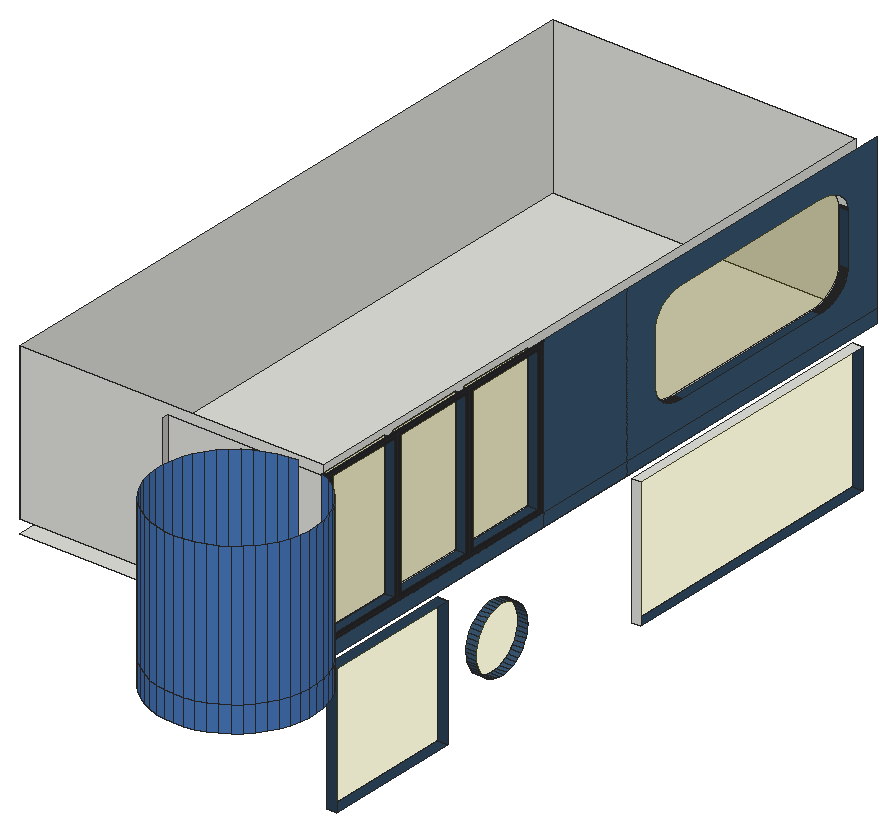
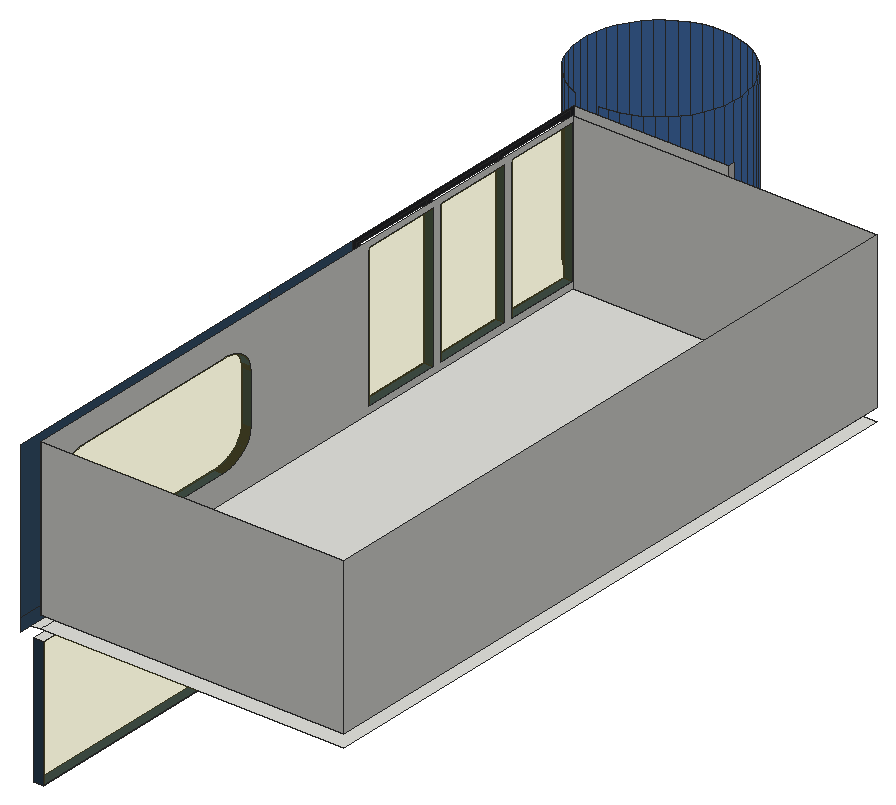
# SketchUp Ruby script. Lengths in inches.
U = 1.inch
M = Sketchup.active_model
def pt(a) = Geom::Point3d.new(a.map { |v| v * U })
def face(e, loops, mat)
  f = e.add_face(loops[0].map { |a| pt(a) })
  loops[1..].each { |l| e.add_face(l.map { |a| pt(a) }).erase! }
  f.material = f.back_material = mat if mat
  f
end
# faces: each face lists its corners as indices into pts; further lists are holes
def faces(e, pts, list, mat = nil) = list.each { |f| face(e, (f[0].is_a?(Array) ? f : [f]).map { |l| l.map { |i| pts[i] } }, mat) }
# xy, xz, yz: faces in a plane at the given z, y or x. An outline is a flat list of corners, or four numbers for a rectangle; further outlines are holes
def ring(l) = l.size == 4 ? [[l[0], l[1]], [l[2], l[1]], [l[2], l[3]], [l[0], l[3]]] : l.each_slice(2).to_a
def flat(e, list, mat, &to3) = list.each { |f| face(e, (f[0].is_a?(Array) ? f : [f]).map { |l| ring(l).map { |u, v| to3.(u, v) } }, mat) }
def xy(e, z, list, mat = nil) = flat(e, list, mat) { |x, y| [x, y, z] }
def xz(e, y, list, mat = nil) = flat(e, list, mat) { |x, z| [x, y, z] }
def yz(e, x, list, mat = nil) = flat(e, list, mat) { |y, z| [x, y, z] }
def lines(e, pts, list) = list.each { |a, b| e.add_line(pt(pts[a]), pt(pts[b])) }
# prism: a flat outline (further loops are holes) pulled along v
def prism(e, loops, v, mat = nil)
  f = face(e, loops, mat); d = Geom::Vector3d.new(v.map { |x| x * U })
  f.pushpull(f.normal.samedirection?(d) ? d.length : -d.length)
end
def box(e, o, s, mat = nil) = prism(e, [[o, [o[0] + s[0], o[1], o[2]], [o[0] + s[0], o[1] + s[1], o[2]], [o[0], o[1] + s[1], o[2]]]], [0, 0, s[2]], mat)
def at(x, y, z, deg = 0) = Geom::Transformation.translation(pt([x, y, z])) * Geom::Transformation.rotation(ORIGIN, Z_AXIS, deg.degrees)
def axes(o, x, y, z) = Geom::Transformation.new([*x, 0, *y, 0, *z, 0, *pt(o).to_a, 1])
def part(name) = M.definitions.add(name)
# library, detail: a bought-in or finely detailed component or shape, given as its bounding box
def library(name, o, s) = part(name).tap { |d| box(d.entities, o, s) }
def detail(e, o, s) = box(e.add_group.entities, o, s)
def put(e, d, t, mat = nil) = e.add_instance(d, t).tap { |i| i.material = mat if mat }
def group(e, t, mat = nil) = e.add_group.tap { |g| g.transformation = t; g.material = mat if mat }.entities
root = M.entities
M.materials.add("Carpet_01_1K").color = [196, 195, 193]
M.materials.add("Carpet_04_1K").color = [56, 85, 112]
M.materials.add("Carpet_04_1K1").color = [43, 65, 85]
M.materials.add("Glass_Basic_01").color = [186, 175, 28]
M.materials["Glass_Basic_01"].alpha = 0.25
M.materials.add("Glass_Mirror_01").color = [71, 118, 185]
M.materials.add("ThomThom - Buttons2").color = [40, 40, 43]
xy(root,12,[[321.57,171.58,330.57,300.22],[321.57,525.34,330.57,782.62]],"Carpet_04_1K1")
xy(root,132,[[321.57,525.34,330.57,782.62]])
xy(root,132,[[321.57,171.58,330.57,300.22]],"Carpet_04_1K1")
xy(root,144,[[321.57,155.5,330.57,786.64],[39.57,167.5625,321.57,786.64]])
xy(root,156,[[39.57,167.5625,321.57,786.64]])
xy(root,162,[[321.57,167.5625,330.57,238.58],[321.57,246.62,330.57,321.66],[321.57,329.7,330.57,404.74]],"Carpet_04_1K1")
xy(root,180,[[321.57,573.58,330.57,734.38]],"Carpet_04_1K1")
xz(root,155.5,[[186.57,144,330.57,156],[186.57,156,330.57,300]])
xz(root,167.5625,[[39.57,156,321.57,300]])
xz(root,167.5625,[[321.57,162,330.57,294]],"Carpet_04_1K1")
xz(root,171.58,[[321.57,12,330.57,132]],"Carpet_04_1K1")
xz(root,238.58,[[321.57,162,330.57,294]],"Carpet_04_1K1")
xz(root,246.62,[[321.57,162,330.57,294]],"Carpet_04_1K1")
xz(root,300.22,[[321.57,12,330.57,132]],"Carpet_04_1K1")
xz(root,321.66,[[321.57,162,330.57,294]],"Carpet_04_1K1")
xz(root,329.7,[[321.57,162,330.57,294]],"Carpet_04_1K1")
xz(root,404.74,[[321.57,162,330.57,294]],"Carpet_04_1K1")
xz(root,525.34,[[321.57,12,330.57,132]])
xz(root,541.42,[[321.57,204,330.57,252]],"Carpet_04_1K1")
xz(root,766.54,[[321.57,204,330.57,252]],"Carpet_04_1K1")
xz(root,782.62,[[321.57,12,330.57,132]],"Carpet_04_1K1")
xz(root,786.64,[[39.57,156,321.57,300]])
yz(root,39.57,[[167.5625,156,786.64,300]])
yz(root,186.57,[[149.51,144,155.5,156],[149.51,156,155.5,300]],"Carpet_01_1K")
yz(root,236.92,[[77.22,150,86.26,174],[77.22,174,86.26,306]],"Glass_Mirror_01")
yz(root,321.57,[[[167.5625,156,167.5625,162,238.58,162,238.58,294,167.5625,294,167.5625,300,786.64,300,786.64,156],[573.58,180,734.38,180,735.39,180.01,736.4,180.05,737.41,180.11,738.41,180.1875,739.41,180.3,740.41,180.43,741.4,180.58,742.38,180.75,743.35,180.95,744.32,181.17,745.27,181.42,746.22,181.69,747.15,181.97,748.07,182.28,748.98,182.62,749.875,182.97,750.75,183.34,751.61,183.74,752.46,184.15,753.28,184.58,754.09,185.04,754.88,185.51,755.65,186,756.4,186.5,757.12,187.03,757.82,187.57,758.5,188.13,759.16,188.7,759.79,189.29,760.4,189.89,760.98,190.51,761.53,191.14,762.0625,191.78,762.5625,192.4375,763.04,193.1,763.48,193.78,763.9,194.47,764.28,195.17,764.64,195.87,764.97,196.58,765.26,197.3,765.53,198.03,765.77,198.76,765.97,199.5,766.14,200.25,766.29,200.99,766.4,201.74,766.48,202.49,766.52,203.25,766.54,204,766.54,252,766.52,252.75,766.48,253.51,766.4,254.26,766.29,255.01,766.14,255.75,765.97,256.5,765.77,257.24,765.53,257.97,765.26,258.7,764.97,259.42,764.64,260.13,764.28,260.83,763.9,261.53,763.48,262.22,763.04,262.9,762.5625,263.5625,762.0625,264.22,761.53,264.86,760.98,265.49,760.4,266.11,759.79,266.71,759.16,267.3,758.5,267.87,757.82,268.43,757.12,268.97,756.4,269.5,755.65,270,754.88,270.49,754.09,270.96,753.28,271.42,752.46,271.85,751.61,272.26,750.75,272.66,749.875,273.03,748.98,273.38,748.07,273.72,747.15,274.03,746.22,274.31,745.27,274.58,744.32,274.83,743.35,275.05,742.38,275.25,741.4,275.42,740.41,275.57,739.41,275.7,738.41,275.8125,737.41,275.89,736.4,275.95,735.39,275.99,734.38,276,573.58,276,572.57,275.99,571.5625,275.95,570.55,275.89,569.55,275.8125,568.55,275.7,567.55,275.57,566.57,275.42,565.58,275.25,564.61,275.05,563.64,274.83,562.6875,274.58,561.74,274.31,560.81,274.03,559.89,273.72,558.98,273.38,558.09,273.03,557.21,272.66,556.35,272.26,555.5,271.85,554.68,271.42,553.87,270.96,553.08,270.49,552.3125,270,551.57,269.5,550.84,268.97,550.14,268.43,549.46,267.87,548.8,267.3,548.17,266.71,547.5625,266.11,546.98,265.49,546.43,264.86,545.9,264.22,545.4,263.5625,544.93,262.9,544.48,262.22,544.07,261.53,543.68,260.83,543.32,260.13,542.99,259.42,542.7,258.7,542.43,257.97,542.2,257.24,541.99,256.5,541.82,255.75,541.67,255.01,541.5625,254.26,541.48,253.51,541.4375,252.75,541.42,252,541.42,204,541.4375,203.25,541.48,202.49,541.5625,201.74,541.67,200.99,541.82,200.25,541.99,199.5,542.2,198.76,542.43,198.03,542.7,197.3,542.99,196.58,543.32,195.87,543.68,195.17,544.07,194.47,544.48,193.78,544.93,193.1,545.4,192.4375,545.9,191.78,546.43,191.14,546.98,190.51,547.5625,189.89,548.17,189.29,548.8,188.7,549.46,188.13,550.14,187.57,550.84,187.03,551.57,186.5,552.3125,186,553.08,185.51,553.87,185.04,554.68,184.58,555.5,184.15,556.35,183.74,557.21,183.34,558.09,182.97,558.98,182.62,559.89,182.28,560.81,181.97,561.74,181.69,562.6875,181.42,563.64,181.17,564.61,180.95,565.58,180.75,566.57,180.58,567.55,180.43,568.55,180.3,569.55,180.1875,570.55,180.11,571.5625,180.05,572.57,180.01],[329.7,162,404.74,294],[246.62,162,321.66,294]]])
yz(root,321.57,[[171.58,12,300.22,132],[525.34,12,782.62,132],[361.46,41.77,357.72,42.22,354.07,43.14,350.5625,44.5,347.25,46.3,344.19,48.5,341.43,51.06,339.01,53.95,336.98,57.125,335.35,60.53,334.17,64.1,333.45,67.8,333.1875,71.56,333.41,75.32,334.09,79.02,335.24,82.61,336.82,86.03,338.82,89.22,341.21,92.14,343.94,94.73,346.98,96.96,350.27,98.79,353.77,100.2,357.41,101.16,361.15,101.65,364.91,101.67,368.65,101.22,372.31,100.3,375.82,98.93,379.13,97.13,382.1875,94.93,384.95,92.37,387.36,89.48,389.4,86.31,391.02,82.91,392.21,79.33,392.93,75.64,393.1875,71.88,392.97,68.12,392.29,64.41,391.14,60.82,389.55,57.41,387.55,54.21,385.17,51.3,382.43,48.7,379.4,46.47,376.11,44.64,372.61,43.24,368.97,42.28,365.23,41.79],[167.5625,162,238.58,294],[246.62,162,321.66,294],
  [329.7,162,404.74,294],[573.58,180,572.57,180.01,571.5625,180.05,570.55,180.11,569.55,180.1875,568.55,180.3,567.55,180.43,566.57,180.58,565.58,180.75,564.61,180.95,563.64,181.17,562.6875,181.42,561.74,181.69,560.81,181.97,559.89,182.28,558.98,182.62,558.09,182.97,557.21,183.34,556.35,183.74,555.5,184.15,554.68,184.58,553.87,185.04,553.08,185.51,552.3125,186,551.57,186.5,550.84,187.03,550.14,187.57,549.46,188.13,548.8,188.7,548.17,189.29,547.5625,189.89,546.98,190.51,546.43,191.14,545.9,191.78,545.4,192.4375,544.93,193.1,544.48,193.78,544.07,194.47,543.68,195.17,543.32,195.87,542.99,196.58,542.7,197.3,542.43,198.03,542.2,198.76,541.99,199.5,541.82,200.25,541.67,200.99,541.5625,201.74,541.48,202.49,541.4375,203.25,541.42,204,541.42,252,541.4375,252.75,541.48,253.51,541.5625,254.26,541.67,255.01,541.82,255.75,541.99,256.5,542.2,257.24,542.43,257.97,542.7,258.7,542.99,259.42,543.32,260.13,543.68,260.83,544.07,261.53,544.48,262.22,544.93,262.9,545.4,263.5625,545.9,264.22,546.43,264.86,546.98,265.49,547.5625,266.11,548.17,266.71,548.8,267.3,549.46,267.87,550.14,268.43,550.84,268.97,551.57,269.5,552.3125,270,553.08,270.49,553.87,270.96,554.68,271.42,555.5,271.85,556.35,272.26,557.21,272.66,558.09,273.03,558.98,273.38,559.89,273.72,560.81,274.03,561.74,274.31,562.6875,274.58,563.64,274.83,564.61,275.05,565.58,275.25,566.57,275.42,567.55,275.57,568.55,275.7,569.55,275.8125,570.55,275.89,571.5625,275.95,572.57,275.99,573.58,276,734.38,276,735.39,275.99,736.4,275.95,737.41,275.89,738.41,275.8125,739.41,275.7,740.41,275.57,741.4,275.42,742.38,275.25,743.35,275.05,744.32,274.83,745.27,274.58,746.22,274.31,747.15,274.03,748.07,273.72,748.98,273.38,749.875,273.03,750.75,272.66,751.61,272.26,752.46,271.85,753.28,271.42,754.09,270.96,754.88,270.49,755.65,270,756.4,269.5,757.12,268.97,757.82,268.43,758.5,267.87,759.16,267.3,759.79,266.71,760.4,266.11,760.98,265.49,761.53,264.86,762.0625,264.22,762.5625,263.5625,763.04,262.9,763.48,262.22,763.9,261.53,764.28,260.83,764.64,260.13,764.97,259.42,765.26,258.7,765.53,257.97,765.77,257.24,765.97,256.5,766.14,255.75,766.29,255.01,766.4,254.26,766.48,253.51,766.52,252.75,766.54,252,766.54,204,766.52,203.25,766.48,202.49,766.4,201.74,766.29,200.99,766.14,200.25,765.97,199.5,765.77,198.76,765.53,198.03,765.26,197.3,764.97,196.58,764.64,195.87,764.28,195.17,763.9,194.47,763.48,193.78,763.04,193.1,762.5625,192.4375,762.0625,191.78,761.53,191.14,760.98,190.51,760.4,189.89,759.79,189.29,759.16,188.7,758.5,188.13,757.82,187.57,757.12,187.03,756.4,186.5,755.65,186,754.88,185.51,754.09,185.04,753.28,184.58,752.46,184.15,751.61,183.74,750.75,183.34,749.875,182.97,748.98,182.62,748.07,182.28,747.15,181.97,746.22,181.69,745.27,181.42,744.32,181.17,743.35,180.95,742.38,180.75,741.4,180.58,740.41,180.43,739.41,180.3,738.41,180.1875,737.41,180.11,736.4,180.05,735.39,180.01,734.38,180]],"Glass_Basic_01")
yz(root,330.57,[[155.5,144,412.78,156],[412.78,144,509.26,156],[509.26,144,798.7,156],[412.78,156,509.26,300],[[509.26,156,798.7,300],[573.58,180,572.57,180.01,571.5625,180.05,570.55,180.11,569.55,180.1875,568.55,180.3,567.55,180.43,566.57,180.58,565.58,180.75,564.61,180.95,563.64,181.17,562.6875,181.42,561.74,181.69,560.81,181.97,559.89,182.28,558.98,182.62,558.09,182.97,557.21,183.34,556.35,183.74,555.5,184.15,554.68,184.58,553.87,185.04,553.08,185.51,552.3125,186,551.57,186.5,550.84,187.03,550.14,187.57,549.46,188.13,548.8,188.7,548.17,189.29,547.5625,189.89,546.98,190.51,546.43,191.14,545.9,191.78,545.4,192.4375,544.93,193.1,544.48,193.78,544.07,194.47,543.68,195.17,543.32,195.87,542.99,196.58,542.7,197.3,542.43,198.03,542.2,198.76,541.99,199.5,541.82,200.25,541.67,200.99,541.5625,201.74,541.48,202.49,541.4375,203.25,541.42,204,541.42,252,541.4375,252.75,541.48,253.51,541.5625,254.26,541.67,255.01,541.82,255.75,541.99,256.5,542.2,257.24,542.43,257.97,542.7,258.7,542.99,259.42,543.32,260.13,543.68,260.83,544.07,261.53,544.48,262.22,544.93,262.9,545.4,263.5625,545.9,264.22,546.43,264.86,546.98,265.49,547.5625,266.11,548.17,266.71,548.8,267.3,549.46,267.87,550.14,268.43,550.84,268.97,551.57,269.5,552.3125,270,553.08,270.49,553.87,270.96,554.68,271.42,555.5,271.85,556.35,272.26,557.21,272.66,558.09,273.03,558.98,273.38,559.89,273.72,560.81,274.03,561.74,274.31,562.6875,274.58,563.64,274.83,564.61,275.05,565.58,275.25,566.57,275.42,567.55,275.57,568.55,275.7,569.55,275.8125,570.55,275.89,571.5625,275.95,572.57,275.99,573.58,276,734.38,276,735.39,275.99,736.4,275.95,737.41,275.89,738.41,275.8125,739.41,275.7,740.41,275.57,741.4,275.42,742.38,275.25,743.35,275.05,744.32,274.83,745.27,274.58,746.22,274.31,747.15,274.03,748.07,273.72,748.98,273.38,749.875,273.03,750.75,272.66,751.61,272.26,752.46,271.85,753.28,271.42,754.09,270.96,754.88,270.49,755.65,270,756.4,269.5,757.12,268.97,757.82,268.43,758.5,267.87,759.16,267.3,759.79,266.71,760.4,266.11,760.98,265.49,761.53,264.86,762.0625,264.22,762.5625,263.5625,763.04,262.9,763.48,262.22,763.9,261.53,764.28,260.83,764.64,260.13,764.97,259.42,765.26,258.7,765.53,257.97,765.77,257.24,765.97,256.5,766.14,255.75,766.29,255.01,766.4,254.26,766.48,253.51,766.52,252.75,766.54,252,766.54,204,766.52,203.25,766.48,202.49,766.4,201.74,766.29,200.99,766.14,200.25,765.97,199.5,765.77,198.76,765.53,198.03,765.26,197.3,764.97,196.58,764.64,195.87,764.28,195.17,763.9,194.47,763.48,193.78,763.04,193.1,762.5625,192.4375,762.0625,191.78,761.53,191.14,760.98,190.51,760.4,189.89,759.79,189.29,759.16,188.7,758.5,188.13,757.82,187.57,757.12,187.03,756.4,186.5,755.65,186,754.88,185.51,754.09,185.04,753.28,184.58,752.46,184.15,751.61,183.74,750.75,183.34,749.875,182.97,748.98,182.62,748.07,182.28,747.15,181.97,746.22,181.69,745.27,181.42,744.32,181.17,743.35,180.95,742.38,180.75,741.4,180.58,740.41,180.43,739.41,180.3,738.41,180.1875,737.41,180.11,736.4,180.05,735.39,180.01,734.38,180]]],"Carpet_04_1K")
yz(root,330.57,[[[155.5,156,412.78,300],[159.52,159,408.76,297]],[[159.52,159,242.6,297],[167.5625,162,238.58,294]],[[242.6,159,325.68,297],[246.62,162,321.66,294]],[[325.68,159,408.76,297],[329.7,162,404.74,294]]],"ThomThom - Buttons2")
yz(root,380.64,[[77.22,150,86.26,174],[77.22,174,86.26,306]],"Glass_Mirror_01")
p = [[330.57,357.72,42.22],[330.57,361.46,41.77],[321.57,361.46,41.77],[321.57,357.72,42.22],[330.57,365.23,41.79],[321.57,365.23,41.79],
  [330.57,368.97,42.28],[321.57,368.97,42.28],[330.57,354.07,43.14],[321.57,354.07,43.14],[330.57,372.61,43.24],[321.57,372.61,43.24],
  [330.57,350.5625,44.5],[321.57,350.5625,44.5],[330.57,376.11,44.64],[321.57,376.11,44.64],[330.57,347.25,46.3],[321.57,347.25,46.3],
  [330.57,379.4,46.47],[321.57,379.4,46.47],[330.57,344.19,48.5],[321.57,344.19,48.5],[330.57,382.43,48.7],[321.57,382.43,48.7],
  [330.57,341.43,51.06],[321.57,341.43,51.06],[330.57,385.17,51.3],[321.57,385.17,51.3],[330.57,339.01,53.95],[321.57,339.01,53.95],
  [330.57,387.55,54.21],[321.57,387.55,54.21],[330.57,336.98,57.125],[321.57,336.98,57.125],[330.57,389.55,57.41],[321.57,389.55,57.41],
  [330.57,335.35,60.53],[321.57,335.35,60.53],[330.57,391.14,60.82],[321.57,391.14,60.82],[330.57,334.17,64.1],[321.57,334.17,64.1],
  [330.57,392.29,64.41],[321.57,392.29,64.41],[330.57,333.45,67.8],[321.57,333.45,67.8],[330.57,392.97,68.12],[321.57,392.97,68.12],
  [330.57,333.1875,71.56],[321.57,333.1875,71.56],[330.57,393.1875,71.88],[321.57,393.1875,71.88],[330.57,333.41,75.32],[321.57,333.41,75.32],
  [330.57,392.93,75.64],[321.57,392.93,75.64],[330.57,334.09,79.02],[321.57,334.09,79.02],[330.57,392.21,79.33],[321.57,392.21,79.33],
  [330.57,335.24,82.61],[321.57,335.24,82.61],[330.57,391.02,82.91],[321.57,391.02,82.91],[330.57,336.82,86.03],[321.57,336.82,86.03],
  [330.57,389.4,86.31],[321.57,389.4,86.31],[330.57,338.82,89.22],[321.57,338.82,89.22],[330.57,387.36,89.48],[321.57,387.36,89.48],
  [330.57,341.21,92.14],[321.57,341.21,92.14],[330.57,384.95,92.37],[321.57,384.95,92.37],[330.57,343.94,94.73],[321.57,343.94,94.73],
  [330.57,382.1875,94.93],[321.57,382.1875,94.93],[330.57,346.98,96.96],[321.57,346.98,96.96],[330.57,379.13,97.13],[321.57,379.13,97.13],
  [330.57,350.27,98.79],[321.57,350.27,98.79],[330.57,375.82,98.93],[321.57,375.82,98.93],[330.57,353.77,100.2],[321.57,353.77,100.2],
  [330.57,372.31,100.3],[321.57,372.31,100.3],[330.57,357.41,101.16],[321.57,357.41,101.16],[330.57,368.65,101.22],[321.57,368.65,101.22],
  [330.57,361.15,101.65],[321.57,361.15,101.65],[330.57,364.91,101.67],[321.57,364.91,101.67],[299.76,10.3,174],[299.76,10.3,150],
  [308.78,9.74,150],[308.78,9.74,174],[317.8,10.3,150],[317.8,10.3,174],[290.875,12,174],[290.875,12,150],
  [326.6875,12,150],[326.6875,12,174],[282.28,14.79,174],[282.28,14.79,150],[335.29,14.79,150],[335.29,14.79,174],
  [274.09,18.64,174],[274.09,18.64,150],[343.47,18.64,150],[343.47,18.64,174],[266.46,23.49,174],[266.46,23.49,150],
  [351.1,23.49,150],[351.1,23.49,174],[259.49,29.25,174],[259.49,29.25,150],[358.07,29.25,150],[358.07,29.25,174],
  [253.3,35.84,174],[253.3,35.84,150],[364.26,35.84,150],[364.26,35.84,174],[247.99,43.16,174],[247.99,43.16,150],
  [369.57,43.16,150],[369.57,43.16,174],[243.63,51.08,174],[243.63,51.08,150],[373.93,51.08,150],[373.93,51.08,174],
  [240.3,59.49,174],[240.3,59.49,150],[377.26,59.49,150],[377.26,59.49,174],[238.06,68.25,174],[238.06,68.25,150],
  [379.51,68.25,150],[379.51,68.25,174],[236.92,77.22,174],[236.92,77.22,150],[380.64,77.22,150],[380.64,77.22,174],
  [238.06,95.23,174],[238.06,95.23,150],[236.92,86.26,150],[236.92,86.26,174],[380.64,86.26,174],[380.64,86.26,150],
  [379.51,95.23,150],[379.51,95.23,174],[240.3,103.99,174],[240.3,103.99,150],[377.26,103.99,150],[377.26,103.99,174],
  [243.63,112.39,174],[243.63,112.39,150],[373.93,112.39,150],[373.93,112.39,174],[247.99,120.32,174],[247.99,120.32,150],
  [369.57,120.32,150],[369.57,120.32,174],[253.3,127.63,174],[253.3,127.63,150],[364.26,127.63,150],[364.26,127.63,174],
  [259.49,134.22,174],[259.49,134.22,150],[358.07,134.22,150],[358.07,134.22,174],[266.46,139.99,174],[266.46,139.99,150],
  [351.1,139.99,150],[351.1,139.99,174],[274.09,144.83,174],[274.09,144.83,150],[343.47,144.83,150],[343.47,144.83,174],
  [282.28,148.68,174],[282.28,148.68,150],[335.29,148.68,150],[335.29,148.68,174],[290.875,151.48,174],[290.875,151.48,150],
  [299.76,153.17,174],[299.76,153.17,150],[308.78,153.74,174],[308.78,153.74,150],[299.76,10.3,306],[308.78,9.74,306],
  [317.8,10.3,306],[290.875,12,306],[326.6875,12,306],[282.28,14.79,306],[335.29,14.79,306],[274.09,18.64,306],
  [343.47,18.64,306],[266.46,23.49,306],[351.1,23.49,306],[259.49,29.25,306],[358.07,29.25,306],[253.3,35.84,306],
  [364.26,35.84,306],[247.99,43.16,306],[369.57,43.16,306],[243.63,51.08,306],[373.93,51.08,306],[240.3,59.49,306],
  [377.26,59.49,306],[238.06,68.25,306],[379.51,68.25,306],[236.92,77.22,306],[380.64,77.22,306],[238.06,95.23,306],
  [236.92,86.26,306],[380.64,86.26,306],[379.51,95.23,306],[240.3,103.99,306],[377.26,103.99,306],[243.63,112.39,306],
  [373.93,112.39,306],[247.99,120.32,306],[369.57,120.32,306],[253.3,127.63,306],[364.26,127.63,306],[259.49,134.22,306],
  [358.07,134.22,306],[266.46,139.99,306],[351.1,139.99,306],[274.09,144.83,306],[343.47,144.83,306],[282.28,148.68,306],
  [335.29,148.68,306],[290.875,151.48,306],[299.76,153.17,306],[308.78,153.74,306],[330.57,570.55,180.11],[330.57,571.5625,180.05],
  [321.57,571.5625,180.05],[321.57,570.55,180.11],[330.57,572.57,180.01],[321.57,572.57,180.01],[330.57,573.58,180],[321.57,573.58,180],
  [330.57,734.38,180],[330.57,735.39,180.01],[321.57,735.39,180.01],[321.57,734.38,180],[330.57,736.4,180.05],[321.57,736.4,180.05],
  [330.57,737.41,180.11],[321.57,737.41,180.11],[330.57,569.55,180.1875],[321.57,569.55,180.1875],[330.57,738.41,180.1875],[321.57,738.41,180.1875],
  [330.57,568.55,180.3],[321.57,568.55,180.3],[330.57,739.41,180.3],[321.57,739.41,180.3],[330.57,567.55,180.43],[321.57,567.55,180.43],
  [330.57,740.41,180.43],[321.57,740.41,180.43],[330.57,566.57,180.58],[321.57,566.57,180.58],[330.57,741.4,180.58],[321.57,741.4,180.58],
  [330.57,565.58,180.75],[321.57,565.58,180.75],[330.57,742.38,180.75],[321.57,742.38,180.75],[330.57,564.61,180.95],[321.57,564.61,180.95],
  [330.57,743.35,180.95],[321.57,743.35,180.95],[330.57,563.64,181.17],[321.57,563.64,181.17],[330.57,744.32,181.17],[321.57,744.32,181.17],
  [330.57,562.6875,181.42],[321.57,562.6875,181.42],[330.57,745.27,181.42],[321.57,745.27,181.42],[330.57,561.74,181.69],[321.57,561.74,181.69],
  [330.57,746.22,181.69],[321.57,746.22,181.69],[330.57,560.81,181.97],[321.57,560.81,181.97],[330.57,747.15,181.97],[321.57,747.15,181.97],
  [330.57,559.89,182.28],[321.57,559.89,182.28],[330.57,748.07,182.28],[321.57,748.07,182.28],[330.57,558.98,182.62],[321.57,558.98,182.62],
  [330.57,748.98,182.62],[321.57,748.98,182.62],[330.57,558.09,182.97],[321.57,558.09,182.97],[330.57,749.875,182.97],[321.57,749.875,182.97],
  [330.57,557.21,183.34],[321.57,557.21,183.34],[330.57,750.75,183.34],[321.57,750.75,183.34],[330.57,556.35,183.74],[321.57,556.35,183.74],
  [330.57,751.61,183.74],[321.57,751.61,183.74],[330.57,555.5,184.15],[321.57,555.5,184.15],[330.57,752.46,184.15],[321.57,752.46,184.15],
  [330.57,554.68,184.58],[321.57,554.68,184.58],[330.57,753.28,184.58],[321.57,753.28,184.58],[330.57,553.87,185.04],[321.57,553.87,185.04],
  [330.57,754.09,185.04],[321.57,754.09,185.04],[330.57,553.08,185.51],[321.57,553.08,185.51],[330.57,754.88,185.51],[321.57,754.88,185.51],
  [330.57,552.3125,186],[321.57,552.3125,186],[330.57,755.65,186],[321.57,755.65,186],[330.57,551.57,186.5],[321.57,551.57,186.5],
  [330.57,756.4,186.5],[321.57,756.4,186.5],[330.57,550.84,187.03],[321.57,550.84,187.03],[330.57,757.12,187.03],[321.57,757.12,187.03],
  [330.57,550.14,187.57],[321.57,550.14,187.57],[330.57,757.82,187.57],[321.57,757.82,187.57],[330.57,549.46,188.13],[321.57,549.46,188.13],
  [330.57,758.5,188.13],[321.57,758.5,188.13],[330.57,548.8,188.7],[321.57,548.8,188.7],[330.57,759.16,188.7],[321.57,759.16,188.7],
  [330.57,548.17,189.29],[321.57,548.17,189.29],[330.57,759.79,189.29],[321.57,759.79,189.29],[330.57,547.5625,189.89],[321.57,547.5625,189.89],
  [330.57,760.4,189.89],[321.57,760.4,189.89],[330.57,546.98,190.51],[321.57,546.98,190.51],[330.57,760.98,190.51],[321.57,760.98,190.51],
  [330.57,546.43,191.14],[321.57,546.43,191.14],[330.57,761.53,191.14],[321.57,761.53,191.14],[330.57,545.9,191.78],[321.57,545.9,191.78],
  [330.57,762.0625,191.78],[321.57,762.0625,191.78],[330.57,545.4,192.4375],[321.57,545.4,192.4375],[330.57,762.5625,192.4375],[321.57,762.5625,192.4375],
  [330.57,544.93,193.1],[321.57,544.93,193.1],[330.57,763.04,193.1],[321.57,763.04,193.1],[330.57,544.48,193.78],[321.57,544.48,193.78],
  [330.57,763.48,193.78],[321.57,763.48,193.78],[330.57,544.07,194.47],[321.57,544.07,194.47],[330.57,763.9,194.47],[321.57,763.9,194.47],
  [330.57,543.68,195.17],[321.57,543.68,195.17],[330.57,764.28,195.17],[321.57,764.28,195.17],[330.57,543.32,195.87],[321.57,543.32,195.87],
  [330.57,764.64,195.87],[321.57,764.64,195.87],[330.57,542.99,196.58],[321.57,542.99,196.58],[330.57,764.97,196.58],[321.57,764.97,196.58],
  [330.57,542.7,197.3],[321.57,542.7,197.3],[330.57,765.26,197.3],[321.57,765.26,197.3],[330.57,542.43,198.03],[321.57,542.43,198.03],
  [330.57,765.53,198.03],[321.57,765.53,198.03],[330.57,542.2,198.76],[321.57,542.2,198.76],[330.57,765.77,198.76],[321.57,765.77,198.76],
  [330.57,541.99,199.5],[321.57,541.99,199.5],[330.57,765.97,199.5],[321.57,765.97,199.5],[330.57,541.82,200.25],[321.57,541.82,200.25],
  [330.57,766.14,200.25],[321.57,766.14,200.25],[330.57,541.67,200.99],[321.57,541.67,200.99],[330.57,766.29,200.99],[321.57,766.29,200.99],
  [330.57,541.5625,201.74],[321.57,541.5625,201.74],[330.57,766.4,201.74],[321.57,766.4,201.74],[330.57,541.48,202.49],[321.57,541.48,202.49],
  [330.57,766.48,202.49],[321.57,766.48,202.49],[330.57,541.4375,203.25],[321.57,541.4375,203.25],[330.57,766.52,203.25],[321.57,766.52,203.25],
  [330.57,541.42,204],[321.57,541.42,204],[330.57,766.54,204],[321.57,766.54,204],[330.57,541.4375,252.75],[330.57,541.42,252],
  [321.57,541.42,252],[321.57,541.4375,252.75],[330.57,766.54,252],[330.57,766.52,252.75],[321.57,766.52,252.75],[321.57,766.54,252],
  [330.57,541.48,253.51],[321.57,541.48,253.51],[330.57,766.48,253.51],[321.57,766.48,253.51],[330.57,541.5625,254.26],[321.57,541.5625,254.26],
  [330.57,766.4,254.26],[321.57,766.4,254.26],[330.57,541.67,255.01],[321.57,541.67,255.01],[330.57,766.29,255.01],[321.57,766.29,255.01],
  [330.57,150.21,174],[330.57,150.21,150]]
faces(root,p,[[0,1,2,3],[1,4,5,2],[4,6,7,5],[8,0,3,9],[6,10,11,7],[12,8,9,13],[10,14,15,11],[16,12,13,17],
  [14,18,19,15],[20,16,17,21],[18,22,23,19],[24,20,21,25],[22,26,27,23],[28,24,25,29],[26,30,31,27],[32,28,29,33],
  [30,34,35,31],[36,32,33,37],[34,38,39,35],[40,36,37,41],[38,42,43,39],[44,40,41,45],[42,46,47,43],[48,44,45,49],
  [46,50,51,47],[52,48,49,53],[50,54,55,51],[56,52,53,57],[54,58,59,55],[60,56,57,61],[58,62,63,59],[64,60,61,65],
  [62,66,67,63],[68,64,65,69],[66,70,71,67],[72,68,69,73],[70,74,75,71],[76,72,73,77],[74,78,79,75],[80,76,77,81],
  [78,82,83,79],[84,80,81,85],[82,86,87,83],[88,84,85,89],[86,90,91,87],[92,88,89,93],[90,94,95,91],[96,92,93,97],
  [94,98,99,95],[98,96,97,99]],"Carpet_04_1K")
faces(root,p,[[100,101,102,103],[103,102,104,105],[106,107,101,100],[105,104,108,109],[110,111,107,106],[109,108,112,113],[114,115,111,110],[113,112,116,117],
  [118,119,115,114],[117,116,120,121],[122,123,119,118],[121,120,124,125],[126,127,123,122],[125,124,128,129],[130,131,127,126],[129,128,132,133],
  [134,135,131,130],[133,132,136,137],[138,139,135,134],[137,136,140,141],[142,143,139,138],[141,140,144,145],[146,147,143,142],[145,144,148,149],
  [150,151,152,153],[154,155,156,157],[158,159,151,150],[157,156,160,161],[162,163,159,158],[161,160,164,165],[166,167,163,162],[165,164,168,169],
  [170,171,167,166],[169,168,172,173],[174,175,171,170],[173,172,176,177],[178,179,175,174],[177,176,180,181],[182,183,179,178],[181,180,184,185],
  [186,187,183,182],[185,184,188,189],[190,191,187,186],[192,193,191,190],[194,195,193,192],[196,100,103,197],[197,103,105,198],[199,106,100,196],
  [198,105,109,200],[201,110,106,199],[200,109,113,202],[203,114,110,201],[202,113,117,204],[205,118,114,203],[204,117,121,206],[207,122,118,205],
  [206,121,125,208],[209,126,122,207],[208,125,129,210],[211,130,126,209],[210,129,133,212],[213,134,130,211],[212,133,137,214],[215,138,134,213],
  [214,137,141,216],[217,142,138,215],[216,141,145,218],[219,146,142,217],[218,145,149,220],[221,150,153,222],[223,154,157,224],[225,158,150,221],
  [224,157,161,226],[227,162,158,225],[226,161,165,228],[229,166,162,227],[228,165,169,230],[231,170,166,229],[230,169,173,232],[233,174,170,231],
  [232,173,177,234],[235,178,174,233],[234,177,181,236],[237,182,178,235],[236,181,185,238],[239,186,182,237],[238,185,189,240],[241,190,186,239],
  [242,192,190,241],[243,194,192,242]],"Glass_Mirror_01")
faces(root,p,[[244,245,246,247],[245,248,249,246],[248,250,251,249],[252,253,254,255],[253,256,257,254],[256,258,259,257],[260,244,247,261],[258,262,263,259],
  [264,260,261,265],[262,266,267,263],[268,264,265,269],[266,270,271,267],[272,268,269,273],[270,274,275,271],[276,272,273,277],[274,278,279,275],
  [280,276,277,281],[278,282,283,279],[284,280,281,285],[282,286,287,283],[288,284,285,289],[286,290,291,287],[292,288,289,293],[290,294,295,291],
  [296,292,293,297],[294,298,299,295],[300,296,297,301],[298,302,303,299],[304,300,301,305],[302,306,307,303],[308,304,305,309],[306,310,311,307],
  [312,308,309,313],[310,314,315,311],[316,312,313,317],[314,318,319,315],[320,316,317,321],[318,322,323,319],[324,320,321,325],[322,326,327,323],
  [328,324,325,329],[326,330,331,327],[332,328,329,333],[330,334,335,331],[336,332,333,337],[334,338,339,335],[340,336,337,341],[338,342,343,339],
  [344,340,341,345],[342,346,347,343],[348,344,345,349],[346,350,351,347],[352,348,349,353],[350,354,355,351],[356,352,353,357],[354,358,359,355],
  [360,356,357,361],[358,362,363,359],[364,360,361,365],[362,366,367,363],[368,364,365,369],[366,370,371,367],[372,368,369,373],[370,374,375,371],
  [376,372,373,377],[374,378,379,375],[380,376,377,381],[378,382,383,379],[384,380,381,385],[382,386,387,383],[388,384,385,389],[386,390,391,387],
  [392,388,389,393],[390,394,395,391],[396,392,393,397],[394,398,399,395],[400,396,397,401],[398,402,403,399],[404,400,401,405],[402,406,407,403],
  [408,404,405,409],[406,410,411,407],[412,408,409,413],[410,414,415,411],[416,412,413,417],[414,418,419,415],[420,416,417,421],[418,422,423,419],
  [424,420,421,425],[422,426,427,423],[428,424,425,429],[426,430,431,427],[432,428,429,433],[430,434,435,431],[436,432,433,437],[434,438,439,435],
  [440,436,437,441],[438,442,443,439],[444,440,441,445],[442,446,447,443],[448,449,450,451],[452,453,454,455],[456,448,451,457],[453,458,459,454],
  [460,456,457,461],[458,462,463,459],[464,460,461,465],[462,466,467,463]],"Carpet_04_1K1")
lines(root,p,[[189,468],[188,469]])
